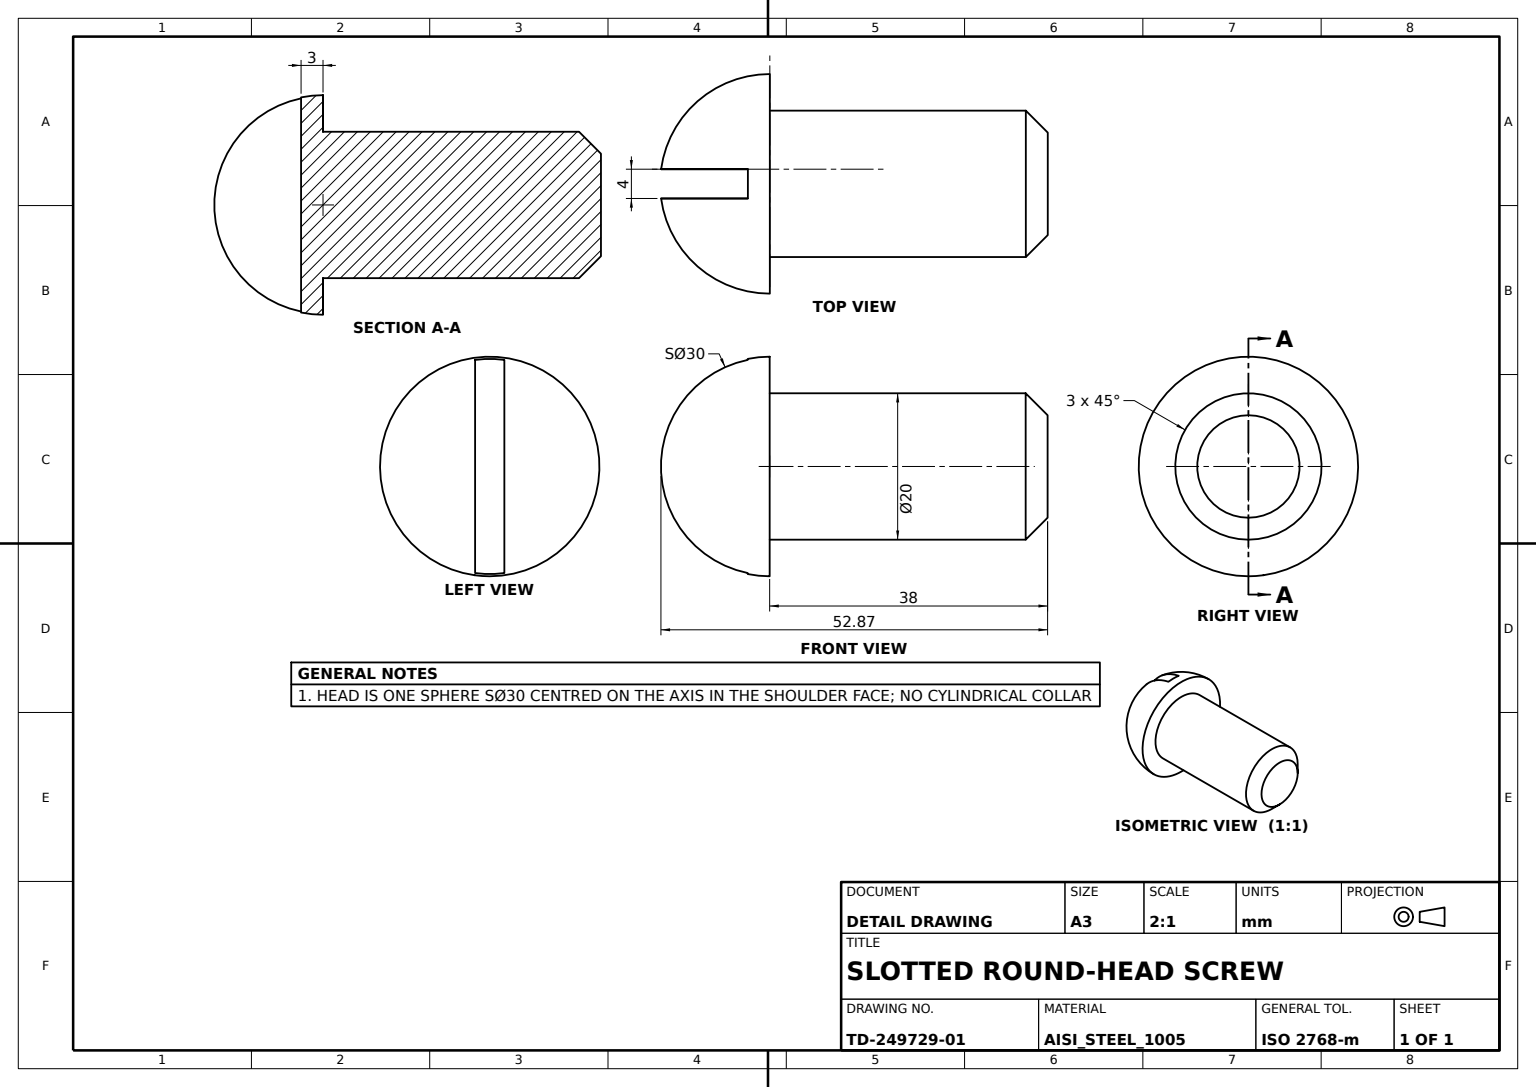
ISO-10303-21;
HEADER;
FILE_DESCRIPTION((''),'2;1');
FILE_NAME('','',(''),(''),'','','');
FILE_SCHEMA(('AUTOMOTIVE_DESIGN'));
ENDSEC;
DATA;
#1=APPLICATION_CONTEXT('');
#2=PRODUCT_CONTEXT('',#1,'mechanical');
#3=PRODUCT('','','',(#2));
#4=PRODUCT_DEFINITION_FORMATION('','',#3);
#5=PRODUCT_DEFINITION_CONTEXT('',#1,'design');
#6=PRODUCT_DEFINITION('','',#4,#5);
#7=PRODUCT_DEFINITION_SHAPE('','',#6);
#8=(LENGTH_UNIT()NAMED_UNIT(*)SI_UNIT(.MILLI.,.METRE.));
#9=(NAMED_UNIT(*)PLANE_ANGLE_UNIT()SI_UNIT($,.RADIAN.));
#10=(NAMED_UNIT(*)SI_UNIT($,.STERADIAN.)SOLID_ANGLE_UNIT());
#11=UNCERTAINTY_MEASURE_WITH_UNIT(LENGTH_MEASURE(0.005),#8,'distance_accuracy_value','');
#12=(GEOMETRIC_REPRESENTATION_CONTEXT(3)GLOBAL_UNCERTAINTY_ASSIGNED_CONTEXT((#11))GLOBAL_UNIT_ASSIGNED_CONTEXT((#8,#9,#10))REPRESENTATION_CONTEXT('',''));
#13=CARTESIAN_POINT('',(-3.,2.,-14.56022));
#14=VERTEX_POINT('',#13);
#15=CARTESIAN_POINT('',(-3.,2.,14.56022));
#16=VERTEX_POINT('',#15);
#17=CARTESIAN_POINT('',(0.,2.,0.));
#18=DIRECTION('',(0.,-1.,0.));
#19=DIRECTION('',(1.,0.,0.));
#20=AXIS2_PLACEMENT_3D('',#17,#18,#19);
#21=CIRCLE('',#20,14.866069);
#22=EDGE_CURVE('',#14,#16,#21,.F.);
#23=ORIENTED_EDGE('',*,*,#22,.F.);
#24=CARTESIAN_POINT('',(-3.,2.,25.));
#25=DIRECTION('',(0.,0.,-1.));
#26=VECTOR('',#25,1000.);
#27=LINE('',#24,#26);
#28=EDGE_CURVE('',#14,#16,#27,.F.);
#29=ORIENTED_EDGE('',*,*,#28,.T.);
#30=EDGE_LOOP('',(#23,#29));
#31=FACE_BOUND('',#30,.T.);
#32=AXIS2_PLACEMENT_3D('',#24,#18,#19);
#33=PLANE('',#32);
#34=ADVANCED_FACE('',(#31),#33,.T.);
#35=CARTESIAN_POINT('',(-3.,-2.,-14.56022));
#36=VERTEX_POINT('',#35);
#37=CARTESIAN_POINT('',(-3.,-2.,14.56022));
#38=VERTEX_POINT('',#37);
#39=CARTESIAN_POINT('',(-3.,-2.,25.));
#40=LINE('',#39,#26);
#41=EDGE_CURVE('',#36,#38,#40,.F.);
#42=ORIENTED_EDGE('',*,*,#41,.T.);
#43=CARTESIAN_POINT('',(-3.,0.,0.));
#44=DIRECTION('',(-1.,0.,0.));
#45=DIRECTION('',(0.,0.,1.));
#46=AXIS2_PLACEMENT_3D('',#43,#44,#45);
#47=CIRCLE('',#46,14.696938);
#48=EDGE_CURVE('',#16,#38,#47,.F.);
#49=ORIENTED_EDGE('',*,*,#48,.F.);
#50=ORIENTED_EDGE('',*,*,#28,.F.);
#51=EDGE_CURVE('',#36,#14,#47,.F.);
#52=ORIENTED_EDGE('',*,*,#51,.F.);
#53=EDGE_LOOP('',(#42,#49,#50,#52));
#54=FACE_BOUND('',#53,.T.);
#55=AXIS2_PLACEMENT_3D('',#39,#44,#45);
#56=PLANE('',#55);
#57=ADVANCED_FACE('',(#54),#56,.T.);
#58=CARTESIAN_POINT('',(0.,0.,-15.));
#59=VERTEX_POINT('',#58);
#60=CARTESIAN_POINT('',(0.,0.,0.));
#61=AXIS2_PLACEMENT_3D('',#60,#19,#25);
#62=CIRCLE('',#61,15.);
#63=EDGE_CURVE('',#59,#59,#62,.T.);
#64=ORIENTED_EDGE('',*,*,#63,.F.);
#65=EDGE_LOOP('',(#64));
#66=FACE_BOUND('',#65,.T.);
#67=ORIENTED_EDGE('',*,*,#48,.T.);
#68=CARTESIAN_POINT('',(0.,-2.,0.));
#69=DIRECTION('',(0.,1.,0.));
#70=AXIS2_PLACEMENT_3D('',#68,#69,#44);
#71=CIRCLE('',#70,14.866069);
#72=EDGE_CURVE('',#38,#36,#71,.F.);
#73=ORIENTED_EDGE('',*,*,#72,.T.);
#74=ORIENTED_EDGE('',*,*,#51,.T.);
#75=ORIENTED_EDGE('',*,*,#22,.T.);
#76=EDGE_LOOP('',(#67,#73,#74,#75));
#77=FACE_BOUND('',#76,.T.);
#78=AXIS2_PLACEMENT_3D('',#60,#19,#69);
#79=SPHERICAL_SURFACE('',#78,15.);
#80=ADVANCED_FACE('',(#66,#77),#79,.T.);
#81=CARTESIAN_POINT('',(0.,0.,-10.));
#82=VERTEX_POINT('',#81);
#83=CIRCLE('',#61,10.);
#84=EDGE_CURVE('',#82,#82,#83,.T.);
#85=ORIENTED_EDGE('',*,*,#84,.F.);
#86=EDGE_LOOP('',(#85));
#87=FACE_BOUND('',#86,.T.);
#88=ORIENTED_EDGE('',*,*,#63,.T.);
#89=EDGE_LOOP('',(#88));
#90=FACE_BOUND('',#89,.T.);
#91=CARTESIAN_POINT('',(0.,10.,0.));
#92=AXIS2_PLACEMENT_3D('',#91,#19,#25);
#93=PLANE('',#92);
#94=ADVANCED_FACE('',(#87,#90),#93,.T.);
#95=ORIENTED_EDGE('',*,*,#84,.T.);
#96=EDGE_LOOP('',(#95));
#97=FACE_BOUND('',#96,.T.);
#98=CARTESIAN_POINT('',(35.,0.,-10.));
#99=VERTEX_POINT('',#98);
#100=CARTESIAN_POINT('',(35.,0.,0.));
#101=AXIS2_PLACEMENT_3D('',#100,#19,#25);
#102=CIRCLE('',#101,10.);
#103=EDGE_CURVE('',#99,#99,#102,.F.);
#104=ORIENTED_EDGE('',*,*,#103,.T.);
#105=EDGE_LOOP('',(#104));
#106=FACE_BOUND('',#105,.T.);
#107=CYLINDRICAL_SURFACE('',#61,10.);
#108=ADVANCED_FACE('',(#97,#106),#107,.T.);
#109=CARTESIAN_POINT('',(38.,0.,-7.));
#110=VERTEX_POINT('',#109);
#111=CARTESIAN_POINT('',(38.,0.,0.));
#112=AXIS2_PLACEMENT_3D('',#111,#19,#25);
#113=CIRCLE('',#112,7.);
#114=EDGE_CURVE('',#110,#110,#113,.T.);
#115=ORIENTED_EDGE('',*,*,#114,.T.);
#116=EDGE_LOOP('',(#115));
#117=FACE_BOUND('',#116,.T.);
#118=PLANE('',#112);
#119=ADVANCED_FACE('',(#117),#118,.T.);
#120=ORIENTED_EDGE('',*,*,#72,.F.);
#121=ORIENTED_EDGE('',*,*,#41,.F.);
#122=EDGE_LOOP('',(#120,#121));
#123=FACE_BOUND('',#122,.T.);
#124=CARTESIAN_POINT('',(-18.,-2.,25.));
#125=AXIS2_PLACEMENT_3D('',#124,#69,#44);
#126=PLANE('',#125);
#127=ADVANCED_FACE('',(#123),#126,.T.);
#128=ORIENTED_EDGE('',*,*,#114,.F.);
#129=EDGE_LOOP('',(#128));
#130=FACE_BOUND('',#129,.T.);
#131=ORIENTED_EDGE('',*,*,#103,.F.);
#132=EDGE_LOOP('',(#131));
#133=FACE_BOUND('',#132,.T.);
#134=AXIS2_PLACEMENT_3D('',#111,#44,#45);
#135=CONICAL_SURFACE('',#134,7.,0.785398163);
#136=ADVANCED_FACE('',(#130,#133),#135,.T.);
#137=CLOSED_SHELL('',(#34,#57,#80,#94,#108,#119,#127,#136));
#138=MANIFOLD_SOLID_BREP('',#137);
#139=ADVANCED_BREP_SHAPE_REPRESENTATION('',(#138),#12);
#140=SHAPE_DEFINITION_REPRESENTATION(#7,#139);
ENDSEC;
END-ISO-10303-21;
